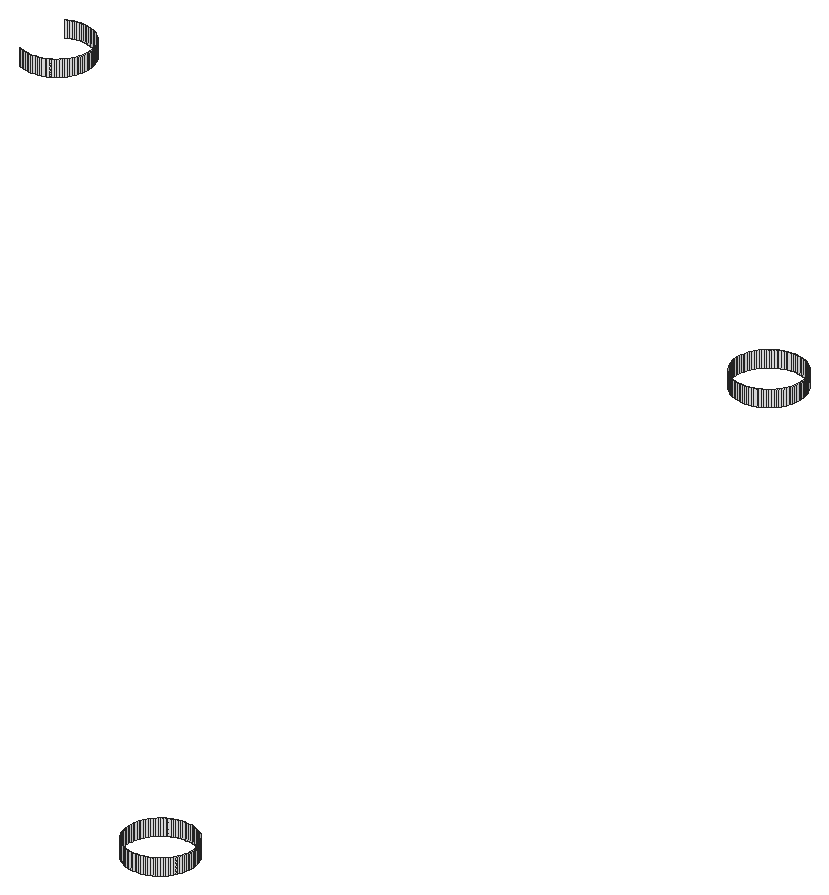
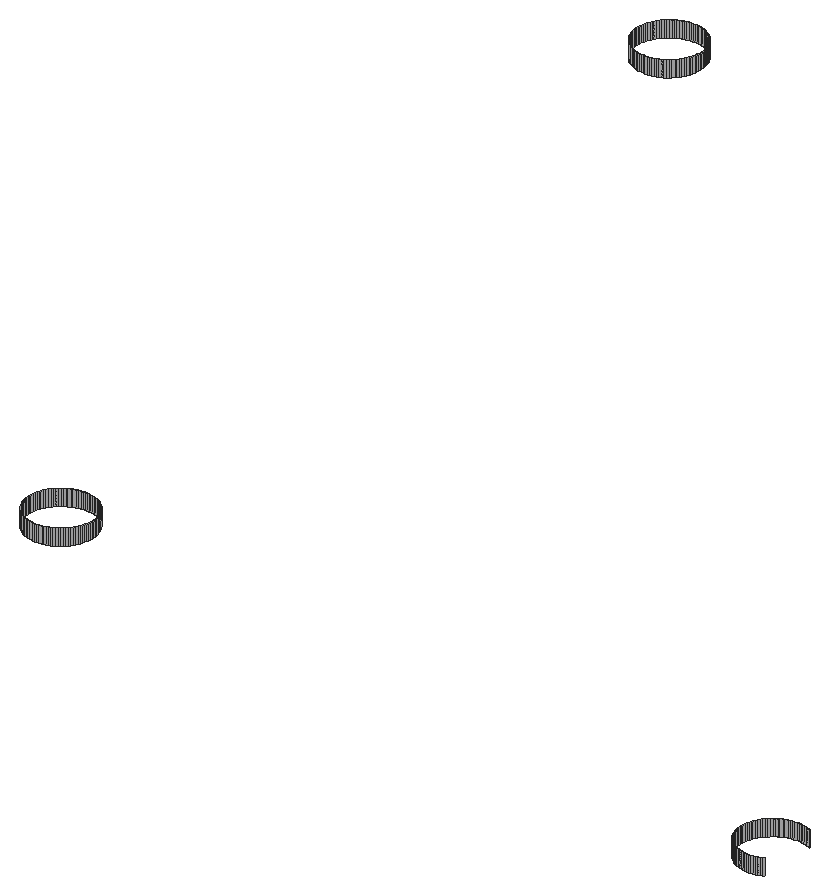
# SketchUp Ruby script. Lengths in inches.
U = 1.inch
M = Sketchup.active_model
def pt(a) = Geom::Point3d.new(a.map { |v| v * U })
def face(e, loops, mat)
  f = e.add_face(loops[0].map { |a| pt(a) })
  loops[1..].each { |l| e.add_face(l.map { |a| pt(a) }).erase! }
  f.material = f.back_material = mat if mat
  f
end
# faces: each face lists its corners as indices into pts; further lists are holes
def faces(e, pts, list, mat = nil) = list.each { |f| face(e, (f[0].is_a?(Array) ? f : [f]).map { |l| l.map { |i| pts[i] } }, mat) }
# xy, xz, yz: faces in a plane at the given z, y or x. An outline is a flat list of corners, or four numbers for a rectangle; further outlines are holes
def ring(l) = l.size == 4 ? [[l[0], l[1]], [l[2], l[1]], [l[2], l[3]], [l[0], l[3]]] : l.each_slice(2).to_a
def flat(e, list, mat, &to3) = list.each { |f| face(e, (f[0].is_a?(Array) ? f : [f]).map { |l| ring(l).map { |u, v| to3.(u, v) } }, mat) }
def xy(e, z, list, mat = nil) = flat(e, list, mat) { |x, y| [x, y, z] }
def xz(e, y, list, mat = nil) = flat(e, list, mat) { |x, z| [x, y, z] }
def yz(e, x, list, mat = nil) = flat(e, list, mat) { |y, z| [x, y, z] }
def lines(e, pts, list) = list.each { |a, b| e.add_line(pt(pts[a]), pt(pts[b])) }
# prism: a flat outline (further loops are holes) pulled along v
def prism(e, loops, v, mat = nil)
  f = face(e, loops, mat); d = Geom::Vector3d.new(v.map { |x| x * U })
  f.pushpull(f.normal.samedirection?(d) ? d.length : -d.length)
end
def box(e, o, s, mat = nil) = prism(e, [[o, [o[0] + s[0], o[1], o[2]], [o[0] + s[0], o[1] + s[1], o[2]], [o[0], o[1] + s[1], o[2]]]], [0, 0, s[2]], mat)
def at(x, y, z, deg = 0) = Geom::Transformation.translation(pt([x, y, z])) * Geom::Transformation.rotation(ORIGIN, Z_AXIS, deg.degrees)
def axes(o, x, y, z) = Geom::Transformation.new([*x, 0, *y, 0, *z, 0, *pt(o).to_a, 1])
def part(name) = M.definitions.add(name)
# library, detail: a bought-in or finely detailed component or shape, given as its bounding box
def library(name, o, s) = part(name).tap { |d| box(d.entities, o, s) }
def detail(e, o, s) = box(e.add_group.entities, o, s)
def put(e, d, t, mat = nil) = e.add_instance(d, t).tap { |i| i.material = mat if mat }
def group(e, t, mat = nil) = e.add_group.tap { |g| g.transformation = t; g.material = mat if mat }.entities
root = M.entities
M.materials.add("[Quartz Light Grey]").color = [251, 251, 252]
xz(root,166.71,[[188.85,111.81,188.98,112.81],[188.98,111.81,189.1,112.81]],"[Quartz Light Grey]")
xz(root,170.71,[[188.9,111.81,189.02,112.81]],"[Quartz Light Grey]")
yz(root,137,[[228.04,111.81,228.17,112.81]],"[Quartz Light Grey]")
yz(root,181,[[223.96,111.81,224.08,112.81]],"[Quartz Light Grey]")
yz(root,185,[[224.04,111.81,224.17,112.81]],"[Quartz Light Grey]")
yz(root,187,[[168.6,111.81,168.73,112.81]],"[Quartz Light Grey]")
yz(root,191,[[168.6875,111.81,168.8125,112.81]],"[Quartz Light Grey]")
p = [[188.6,166.75,111.81],[188.48,166.78,111.81],[188.48,166.78,112.81],[188.6,166.75,112.81],[188.73,166.73,111.81],[188.73,166.73,112.81],
  [188.85,166.71,111.81],[188.85,166.71,112.81],[189.23,166.72,111.81],[189.1,166.71,111.81],[189.1,166.71,112.81],[189.23,166.72,112.81],
  [189.35,166.74,111.81],[189.35,166.74,112.81],[189.48,166.77,111.81],[189.48,166.77,112.81],[188.36,166.8125,111.81],[188.24,166.86,111.81],
  [188.24,166.86,112.81],[188.36,166.8125,112.81],[189.6,166.8,111.81],[189.6,166.8,112.81],[189.72,166.84,111.81],[189.72,166.84,112.81],
  [189.83,166.89,111.81],[189.83,166.89,112.81],[188.13,166.91,111.81],[188.02,166.97,111.81],[188.02,166.97,112.81],[188.13,166.91,112.81],
  [189.94,166.95,111.81],[189.94,166.95,112.81],[190.05,167.01,111.81],[190.05,167.01,112.81],[187.91,167.03,111.81],[187.81,167.1,111.81],
  [187.81,167.1,112.81],[187.91,167.03,112.81],[190.16,167.08,111.81],[190.16,167.08,112.81],[187.71,167.18,111.81],[187.71,167.18,112.81],
  [190.26,167.15,111.81],[190.26,167.15,112.81],[187.62,167.27,111.81],[187.62,167.27,112.81],[190.35,167.24,111.81],[190.35,167.24,112.81],
  [190.44,167.32,111.81],[190.44,167.32,112.81],[187.53,167.36,111.81],[187.53,167.36,112.81],[190.53,167.42,111.81],[190.53,167.42,112.81],
  [187.45,167.45,111.81],[187.45,167.45,112.81],[190.61,167.52,111.81],[190.61,167.52,112.81],[187.37,167.55,111.81],[187.37,167.55,112.81],
  [190.68,167.62,111.81],[190.68,167.62,112.81],[187.3,167.66,111.81],[187.3,167.66,112.81],[190.74,167.73,111.81],[190.74,167.73,112.81],
  [187.24,167.76,111.81],[187.24,167.76,112.81],[190.8,167.84,111.81],[190.8,167.84,112.81],[187.18,167.875,111.81],[187.18,167.875,112.81],
  [190.85,167.95,111.81],[190.85,167.95,112.81],[187.13,167.99,111.81],[187.13,167.99,112.81],[187.09,168.11,111.81],[187.09,168.11,112.81],
  [190.9,168.07,111.81],[190.9,168.07,112.81],[187.06,168.23,111.81],[187.06,168.23,112.81],[190.93,168.19,111.81],[190.93,168.19,112.81],
  [187.03,168.35,111.81],[187.03,168.35,112.81],[190.96,168.3125,111.81],[190.96,168.3125,112.81],[190.98,168.4375,111.81],[190.98,168.4375,112.81],
  [187.01,168.48,111.81],[187.01,168.48,112.81],[190.99,168.5625,111.81],[190.99,168.5625,112.81],[187,168.6,111.81],[187,168.6,112.81],
  [191,168.6875,111.81],[191,168.6875,112.81],[187,168.73,111.81],[187.01,168.86,111.81],[187.01,168.86,112.81],[187,168.73,112.81],
  [190.99,168.9375,111.81],[191,168.8125,111.81],[191,168.8125,112.81],[190.99,168.9375,112.81],[187.02,168.98,111.81],[187.02,168.98,112.81],
  [190.97,169.0625,111.81],[190.97,169.0625,112.81],[187.04,169.1,111.81],[187.04,169.1,112.81],[187.07,169.23,111.81],[187.07,169.23,112.81],
  [190.94,169.19,111.81],[190.94,169.19,112.81],[187.1,169.35,111.81],[187.1,169.35,112.81],[190.91,169.31,111.81],[190.91,169.31,112.81],
  [187.15,169.46,111.81],[187.15,169.46,112.81],[190.87,169.42,111.81],[190.87,169.42,112.81],[190.82,169.54,111.81],[190.82,169.54,112.81],
  [187.2,169.58,111.81],[187.2,169.58,112.81],[190.76,169.65,111.81],[190.76,169.65,112.81],[187.26,169.69,111.81],[187.26,169.69,112.81],
  [187.32,169.8,111.81],[187.32,169.8,112.81],[190.7,169.76,111.81],[190.7,169.76,112.81],[187.39,169.9,111.81],[187.39,169.9,112.81],
  [190.63,169.87,111.81],[190.63,169.87,112.81],[187.47,170,111.81],[187.47,170,112.81],[190.55,169.97,111.81],[190.55,169.97,112.81],
  [187.56,170.09,111.81],[187.56,170.09,112.81],[190.47,170.0625,111.81],[190.47,170.0625,112.81],[187.65,170.18,111.81],[187.65,170.18,112.81],
  [190.38,170.15,111.81],[190.38,170.15,112.81],[187.74,170.26,111.81],[187.74,170.26,112.81],[190.19,170.3125,111.81],[190.29,170.24,111.81],
  [190.29,170.24,112.81],[190.19,170.3125,112.81],[187.84,170.34,111.81],[187.84,170.34,112.81],[187.95,170.41,111.81],[187.95,170.41,112.81],
  [190.09,170.39,111.81],[190.09,170.39,112.81],[188.06,170.47,111.81],[188.06,170.47,112.81],[189.98,170.45,111.81],[189.98,170.45,112.81],
  [188.17,170.53,111.81],[188.17,170.53,112.81],[188.28,170.58,111.81],[188.28,170.58,112.81],[189.76,170.56,111.81],[189.87,170.51,111.81],
  [189.87,170.51,112.81],[189.76,170.56,112.81],[188.4,170.62,111.81],[188.4,170.62,112.81],[188.52,170.65,111.81],[188.52,170.65,112.81],
  [189.4,170.67,111.81],[189.52,170.64,111.81],[189.52,170.64,112.81],[189.4,170.67,112.81],[189.64,170.6,111.81],[189.64,170.6,112.81],
  [188.65,170.68,111.81],[188.65,170.68,112.81],[188.77,170.7,111.81],[188.77,170.7,112.81],[188.9,170.71,111.81],[188.9,170.71,112.81],
  [189.02,170.71,111.81],[189.15,170.7,111.81],[189.15,170.7,112.81],[189.02,170.71,112.81],[189.27,170.69,111.81],[189.27,170.69,112.81],
  [182.48,222.13,111.81],[182.36,222.17,111.81],[182.36,222.17,112.81],[182.48,222.13,112.81],[182.6,222.1,111.81],[182.6,222.1,112.81],
  [182.73,222.08,111.81],[182.73,222.08,112.81],[182.85,222.07,111.81],[182.85,222.07,112.81],[182.98,222.0625,111.81],[182.98,222.0625,112.81],
  [183.1,222.07,111.81],[183.1,222.07,112.81],[183.23,222.08,111.81],[183.23,222.08,112.81],[183.35,222.09,111.81],[183.35,222.09,112.81],
  [183.48,222.12,111.81],[183.48,222.12,112.81],[183.6,222.15,111.81],[183.6,222.15,112.81],[182.24,222.21,111.81],[182.13,222.26,111.81],
  [182.13,222.26,112.81],[182.24,222.21,112.81],[183.72,222.2,111.81],[183.72,222.2,112.81],[183.83,222.24,111.81],[183.83,222.24,112.81],
  [183.94,222.3,111.81],[183.94,222.3,112.81],[182.02,222.32,111.81],[181.91,222.39,111.81],[181.91,222.39,112.81],[182.02,222.32,112.81],
  [184.05,222.36,111.81],[184.05,222.36,112.81],[181.81,222.46,111.81],[181.81,222.46,112.81],[184.16,222.43,111.81],[184.16,222.43,112.81],
  [184.26,222.51,111.81],[184.26,222.51,112.81],[181.71,222.54,111.81],[181.62,222.62,111.81],[181.62,222.62,112.81],[181.71,222.54,112.81],
  [184.35,222.59,111.81],[184.35,222.59,112.81],[181.53,222.71,111.81],[181.53,222.71,112.81],[184.44,222.68,111.81],[184.44,222.68,112.81],
  [181.45,222.8,111.81],[181.45,222.8,112.81],[184.53,222.77,111.81],[184.53,222.77,112.81],[181.37,222.9,111.81],[181.37,222.9,112.81],
  [184.61,222.87,111.81],[184.61,222.87,112.81],[181.3,223.01,111.81],[181.3,223.01,112.81],[184.68,222.97,111.81],[184.68,222.97,112.81],
  [181.24,223.12,111.81],[181.24,223.12,112.81],[184.74,223.08,111.81],[184.74,223.08,112.81],[181.18,223.23,111.81],[181.18,223.23,112.81],
  [184.8,223.19,111.81],[184.8,223.19,112.81],[181.13,223.35,111.81],[181.13,223.35,112.81],[184.85,223.31,111.81],[184.85,223.31,112.81],
  [181.09,223.47,111.81],[181.09,223.47,112.81],[184.9,223.42,111.81],[184.9,223.42,112.81],[184.93,223.54,111.81],[184.93,223.54,112.81],
  [181.06,223.59,111.81],[181.06,223.59,112.81],[184.96,223.67,111.81],[184.96,223.67,112.81],[181.03,223.71,111.81],[181.03,223.71,112.81],
  [181.01,223.83,111.81],[181.01,223.83,112.81],[184.98,223.79,111.81],[184.98,223.79,112.81],[181,223.96,111.81],[181,223.96,112.81],
  [184.99,223.92,111.81],[184.99,223.92,112.81],[185,224.04,111.81],[185,224.04,112.81],[181,224.08,111.81],[181.01,224.21,111.81],
  [181.01,224.21,112.81],[181,224.08,112.81],[181.02,224.33,111.81],[181.02,224.33,112.81],[184.99,224.29,111.81],[185,224.17,111.81],
  [185,224.17,112.81],[184.99,224.29,112.81],[181.04,224.46,111.81],[181.04,224.46,112.81],[184.97,224.42,111.81],[184.97,224.42,112.81],
  [184.94,224.54,111.81],[184.94,224.54,112.81],[181.07,224.58,111.81],[181.07,224.58,112.81],[184.91,224.66,111.81],[184.91,224.66,112.81],
  [181.1,224.7,111.81],[181.1,224.7,112.81],[181.15,224.82,111.81],[181.15,224.82,112.81],[184.87,224.78,111.81],[184.87,224.78,112.81],
  [181.2,224.93,111.81],[181.2,224.93,112.81],[184.82,224.89,111.81],[184.82,224.89,112.81],[181.26,225.05,111.81],[181.26,225.05,112.81],
  [184.76,225.01,111.81],[184.76,225.01,112.81],[181.32,225.15,111.81],[181.32,225.15,112.81],[184.7,225.12,111.81],[184.7,225.12,112.81],
  [184.63,225.22,111.81],[184.63,225.22,112.81],[181.39,225.26,111.81],[181.39,225.26,112.81],[184.55,225.32,111.81],[184.55,225.32,112.81],
  [181.47,225.35,111.81],[181.47,225.35,112.81],[184.47,225.42,111.81],[184.47,225.42,112.81],[181.56,225.45,111.81],[181.56,225.45,112.81],
  [181.65,225.54,111.81],[181.65,225.54,112.81],[184.38,225.51,111.81],[184.38,225.51,112.81],[181.74,225.62,111.81],[181.74,225.62,112.81],
  [184.29,225.59,111.81],[184.29,225.59,112.81],[181.84,225.69,111.81],[181.84,225.69,112.81],[184.19,225.67,111.81],[184.19,225.67,112.81],
  [181.95,225.76,111.81],[181.95,225.76,112.81],[183.98,225.8,111.81],[184.09,225.74,111.81],[184.09,225.74,112.81],[183.98,225.8,112.81],
  [182.06,225.83,111.81],[182.06,225.83,112.81],[182.17,225.88,111.81],[182.17,225.88,112.81],[183.87,225.86,111.81],[183.87,225.86,112.81],
  [182.28,225.93,111.81],[182.28,225.93,112.81],[182.4,225.97,111.81],[182.4,225.97,112.81],[183.64,225.96,111.81],[183.76,225.91,111.81],
  [183.76,225.91,112.81],[183.64,225.96,112.81],[182.52,226.01,111.81],[182.52,226.01,112.81],[182.65,226.03,111.81],[182.65,226.03,112.81],
  [182.77,226.05,111.81],[182.77,226.05,112.81],[182.9,226.06,111.81],[182.9,226.06,112.81],[183.15,226.06,111.81],[183.27,226.04,111.81],
  [183.27,226.04,112.81],[183.15,226.06,112.81],[183.4,226.02,111.81],[183.4,226.02,112.81],[183.52,225.99,111.81],[183.52,225.99,112.81],
  [134.48,226.13,111.81],[134.36,226.17,111.81],[134.36,226.17,112.81],[134.48,226.13,112.81],[134.6,226.1,111.81],[134.6,226.1,112.81],
  [134.73,226.08,111.81],[134.73,226.08,112.81],[134.85,226.07,111.81],[134.85,226.07,112.81],[134.98,226.0625,111.81],[134.98,226.0625,112.81],
  [135.1,226.07,111.81],[135.1,226.07,112.81],[135.23,226.08,111.81],[135.23,226.08,112.81],[135.35,226.09,111.81],[135.35,226.09,112.81],
  [135.48,226.12,111.81],[135.48,226.12,112.81],[135.6,226.15,111.81],[135.6,226.15,112.81],[183.02,226.0625,111.81],[183.02,226.0625,112.81],
  [134.24,226.21,111.81],[134.13,226.26,111.81],[134.13,226.26,112.81],[134.24,226.21,112.81],[135.72,226.2,111.81],[135.72,226.2,112.81],
  [135.83,226.24,111.81],[135.83,226.24,112.81],[135.94,226.3,111.81],[135.94,226.3,112.81],[136.05,226.36,111.81],[136.05,226.36,112.81],
  [136.16,226.43,111.81],[136.16,226.43,112.81],[136.26,226.51,111.81],[136.26,226.51,112.81],[136.35,226.59,111.81],[136.35,226.59,112.81],
  [136.44,226.68,111.81],[136.44,226.68,112.81],[136.53,226.77,111.81],[136.53,226.77,112.81],[136.61,226.87,111.81],[136.61,226.87,112.81],
  [136.68,226.97,111.81],[136.68,226.97,112.81],[136.74,227.08,111.81],[136.74,227.08,112.81],[136.8,227.19,111.81],[136.8,227.19,112.81],
  [136.85,227.31,111.81],[136.85,227.31,112.81],[136.9,227.42,111.81],[136.9,227.42,112.81],[136.93,227.54,111.81],[136.93,227.54,112.81],
  [136.96,227.67,111.81],[136.96,227.67,112.81],[136.98,227.79,111.81],[136.98,227.79,112.81],[136.99,227.92,111.81],[136.99,227.92,112.81],
  [137,228.04,111.81],[137,228.04,112.81],[136.99,228.29,111.81],[137,228.17,111.81],[137,228.17,112.81],[136.99,228.29,112.81],
  [136.97,228.42,111.81],[136.97,228.42,112.81],[136.94,228.54,111.81],[136.94,228.54,112.81],[136.91,228.66,111.81],[136.91,228.66,112.81],
  [136.87,228.78,111.81],[136.87,228.78,112.81],[136.82,228.89,111.81],[136.82,228.89,112.81],[136.76,229.01,111.81],[136.76,229.01,112.81],
  [136.7,229.12,111.81],[136.7,229.12,112.81],[136.63,229.22,111.81],[136.63,229.22,112.81],[136.55,229.32,111.81],[136.55,229.32,112.81],
  [136.47,229.42,111.81],[136.47,229.42,112.81],[136.38,229.51,111.81],[136.38,229.51,112.81],[136.29,229.59,111.81],[136.29,229.59,112.81],
  [136.19,229.67,111.81],[136.19,229.67,112.81],[135.98,229.8,111.81],[136.09,229.74,111.81],[136.09,229.74,112.81],[135.98,229.8,112.81],
  [134.06,229.83,111.81],[134.17,229.88,111.81],[134.17,229.88,112.81],[134.06,229.83,112.81],[135.87,229.86,111.81],[135.87,229.86,112.81],
  [134.28,229.93,111.81],[134.28,229.93,112.81],[134.4,229.97,111.81],[134.4,229.97,112.81],[135.64,229.96,111.81],[135.76,229.91,111.81],
  [135.76,229.91,112.81],[135.64,229.96,112.81],[134.52,230.01,111.81],[134.52,230.01,112.81],[134.65,230.03,111.81],[134.65,230.03,112.81],
  [134.77,230.05,111.81],[134.77,230.05,112.81],[134.9,230.06,111.81],[134.9,230.06,112.81],[135.15,230.06,111.81],[135.27,230.04,111.81],
  [135.27,230.04,112.81],[135.15,230.06,112.81],[135.4,230.02,111.81],[135.4,230.02,112.81],[135.52,229.99,111.81],[135.52,229.99,112.81],
  [135.02,230.0625,111.81],[135.02,230.0625,112.81]]
faces(root,p,[[0,1,2,3],[4,0,3,5],[6,4,5,7],[8,9,10,11],[12,8,11,13],[14,12,13,15],[16,17,18,19],[1,16,19,2],
  [20,14,15,21],[22,20,21,23],[24,22,23,25],[26,27,28,29],[17,26,29,18],[30,24,25,31],[32,30,31,33],[34,35,36,37],
  [27,34,37,28],[38,32,33,39],[35,40,41,36],[42,38,39,43],[40,44,45,41],[46,42,43,47],[48,46,47,49],[44,50,51,45],
  [52,48,49,53],[50,54,55,51],[56,52,53,57],[54,58,59,55],[60,56,57,61],[58,62,63,59],[64,60,61,65],[62,66,67,63],
  [68,64,65,69],[66,70,71,67],[72,68,69,73],[70,74,75,71],[74,76,77,75],[78,72,73,79],[76,80,81,77],[82,78,79,83],
  [80,84,85,81],[86,82,83,87],[88,86,87,89],[84,90,91,85],[92,88,89,93],[90,94,95,91],[96,92,93,97],[98,99,100,101],
  [102,103,104,105],[99,106,107,100],[108,102,105,109],[106,110,111,107],[110,112,113,111],[114,108,109,115],[112,116,117,113],[118,114,115,119],
  [116,120,121,117],[122,118,119,123],[124,122,123,125],[120,126,127,121],[128,124,125,129],[126,130,131,127],[130,132,133,131],[134,128,129,135],
  [132,136,137,133],[138,134,135,139],[136,140,141,137],[142,138,139,143],[140,144,145,141],[146,142,143,147],[144,148,149,145],[150,146,147,151],
  [148,152,153,149],[154,155,156,157],[155,150,151,156],[152,158,159,153],[158,160,161,159],[162,154,157,163],[160,164,165,161],[166,162,163,167],
  [164,168,169,165],[168,170,171,169],[172,173,174,175],[173,166,167,174],[170,176,177,171],[176,178,179,177],[180,181,182,183],[181,184,185,182],
  [184,172,175,185],[178,186,187,179],[186,188,189,187],[188,190,191,189],[192,193,194,195],[193,196,197,194],[196,180,183,197],[198,199,200,201],
  [202,198,201,203],[204,202,203,205],[206,204,205,207],[208,206,207,209],[210,208,209,211],[212,210,211,213],[214,212,213,215],[216,214,215,217],
  [218,216,217,219],[220,221,222,223],[199,220,223,200],[224,218,219,225],[226,224,225,227],[228,226,227,229],[230,231,232,233],[221,230,233,222],
  [234,228,229,235],[231,236,237,232],[238,234,235,239],[240,238,239,241],[242,243,244,245],[236,242,245,237],[246,240,241,247],[243,248,249,244],
  [250,246,247,251],[248,252,253,249],[254,250,251,255],[252,256,257,253],[258,254,255,259],[256,260,261,257],[262,258,259,263],[260,264,265,261],
  [266,262,263,267],[264,268,269,265],[270,266,267,271],[268,272,273,269],[274,270,271,275],[272,276,277,273],[278,274,275,279],[280,278,279,281],
  [276,282,283,277],[284,280,281,285],[282,286,287,283],[286,288,289,287],[290,284,285,291],[288,292,293,289],[294,290,291,295],[296,294,295,297],
  [298,299,300,301],[299,302,303,300],[304,305,306,307],[302,308,309,303],[310,304,307,311],[312,310,311,313],[308,314,315,309],[316,312,313,317],
  [314,318,319,315],[318,320,321,319],[322,316,317,323],[320,324,325,321],[326,322,323,327],[324,328,329,325],[330,326,327,331],[328,332,333,329],
  [334,330,331,335],[336,334,335,337],[332,338,339,333],[340,336,337,341],[338,342,343,339],[344,340,341,345],[342,346,347,343],[346,348,349,347],
  [350,344,345,351],[348,352,353,349],[354,350,351,355],[352,356,357,353],[358,354,355,359],[356,360,361,357],[362,363,364,365],[363,358,359,364],
  [360,366,367,361],[366,368,369,367],[370,362,365,371],[368,372,373,369],[372,374,375,373],[376,377,378,379],[377,370,371,378],[374,380,381,375],
  [380,382,383,381],[382,384,385,383],[384,386,387,385],[388,389,390,391],[389,392,393,390],[392,394,395,393],[394,376,379,395],[396,397,398,399],
  [400,396,399,401],[402,400,401,403],[404,402,403,405],[406,404,405,407],[408,406,407,409],[410,408,409,411],[412,410,411,413],[414,412,413,415],
  [416,414,415,417],[386,418,419,387],[418,388,391,419],[420,421,422,423],[397,420,423,398],[424,416,417,425],[426,424,425,427],[428,426,427,429],
  [430,428,429,431],[432,430,431,433],[434,432,433,435],[436,434,435,437],[438,436,437,439],[440,438,439,441],[442,440,441,443],[444,442,443,445],
  [446,444,445,447],[448,446,447,449],[450,448,449,451],[452,450,451,453],[454,452,453,455],[456,454,455,457],[458,456,457,459],[460,458,459,461],
  [462,460,461,463],[464,465,466,467],[468,464,467,469],[470,468,469,471],[472,470,471,473],[474,472,473,475],[476,474,475,477],[478,476,477,479],
  [480,478,479,481],[482,480,481,483],[484,482,483,485],[486,484,485,487],[488,486,487,489],[490,488,489,491],[492,490,491,493],[494,495,496,497],
  [495,492,493,496],[498,499,500,501],[502,494,497,503],[499,504,505,500],[504,506,507,505],[508,509,510,511],[509,502,503,510],[506,512,513,507],
  [512,514,515,513],[514,516,517,515],[516,518,519,517],[520,521,522,523],[521,524,525,522],[524,526,527,525],[526,508,511,527],[518,528,529,519],
  [528,520,523,529]],"[Quartz Light Grey]")
